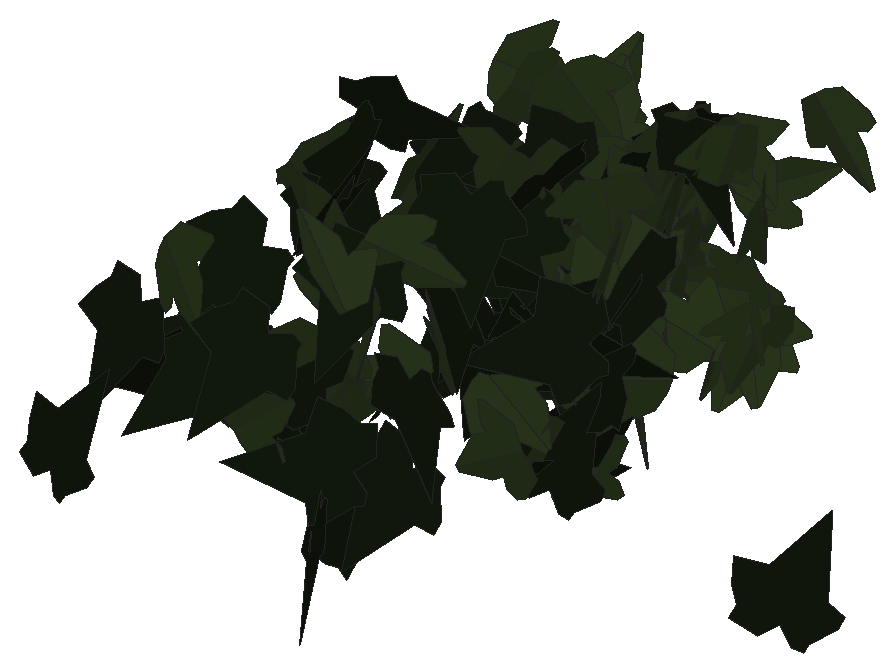
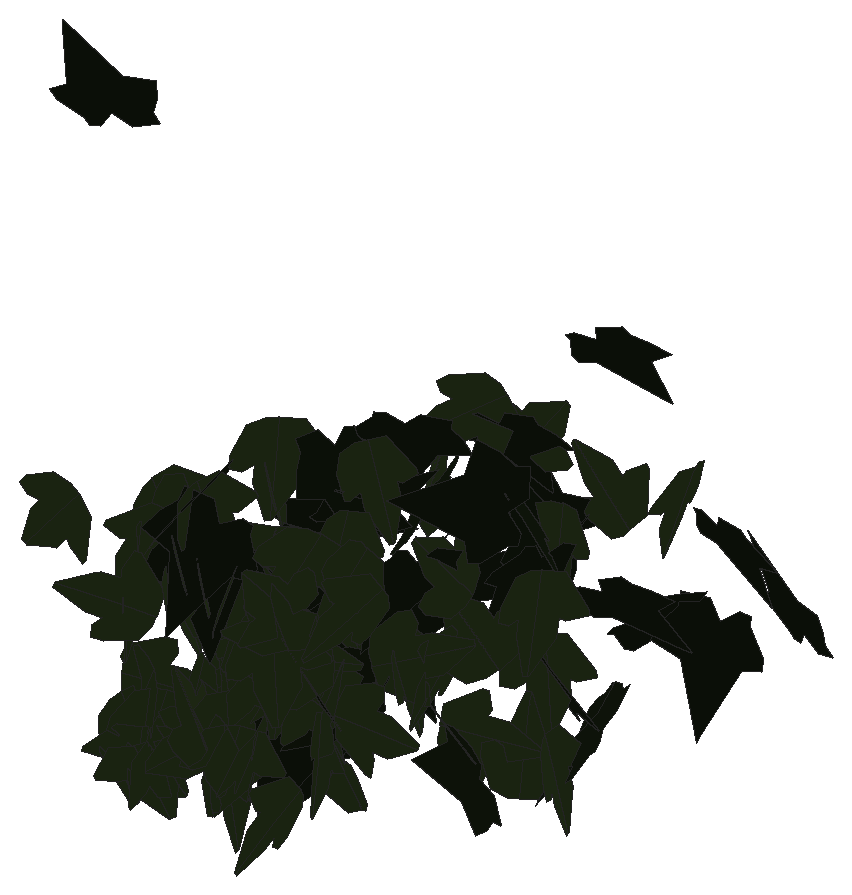
# SketchUp Ruby script. Lengths in inches.
U = 1.inch
M = Sketchup.active_model
def pt(a) = Geom::Point3d.new(a.map { |v| v * U })
def face(e, loops, mat)
  f = e.add_face(loops[0].map { |a| pt(a) })
  loops[1..].each { |l| e.add_face(l.map { |a| pt(a) }).erase! }
  f.material = f.back_material = mat if mat
  f
end
# faces: each face lists its corners as indices into pts; further lists are holes
def faces(e, pts, list, mat = nil) = list.each { |f| face(e, (f[0].is_a?(Array) ? f : [f]).map { |l| l.map { |i| pts[i] } }, mat) }
# xy, xz, yz: faces in a plane at the given z, y or x. An outline is a flat list of corners, or four numbers for a rectangle; further outlines are holes
def ring(l) = l.size == 4 ? [[l[0], l[1]], [l[2], l[1]], [l[2], l[3]], [l[0], l[3]]] : l.each_slice(2).to_a
def flat(e, list, mat, &to3) = list.each { |f| face(e, (f[0].is_a?(Array) ? f : [f]).map { |l| ring(l).map { |u, v| to3.(u, v) } }, mat) }
def xy(e, z, list, mat = nil) = flat(e, list, mat) { |x, y| [x, y, z] }
def xz(e, y, list, mat = nil) = flat(e, list, mat) { |x, z| [x, y, z] }
def yz(e, x, list, mat = nil) = flat(e, list, mat) { |y, z| [x, y, z] }
def lines(e, pts, list) = list.each { |a, b| e.add_line(pt(pts[a]), pt(pts[b])) }
# prism: a flat outline (further loops are holes) pulled along v
def prism(e, loops, v, mat = nil)
  f = face(e, loops, mat); d = Geom::Vector3d.new(v.map { |x| x * U })
  f.pushpull(f.normal.samedirection?(d) ? d.length : -d.length)
end
def box(e, o, s, mat = nil) = prism(e, [[o, [o[0] + s[0], o[1], o[2]], [o[0] + s[0], o[1] + s[1], o[2]], [o[0], o[1] + s[1], o[2]]]], [0, 0, s[2]], mat)
def at(x, y, z, deg = 0) = Geom::Transformation.translation(pt([x, y, z])) * Geom::Transformation.rotation(ORIGIN, Z_AXIS, deg.degrees)
def axes(o, x, y, z) = Geom::Transformation.new([*x, 0, *y, 0, *z, 0, *pt(o).to_a, 1])
def part(name) = M.definitions.add(name)
# library, detail: a bought-in or finely detailed component or shape, given as its bounding box
def library(name, o, s) = part(name).tap { |d| box(d.entities, o, s) }
def detail(e, o, s) = box(e.add_group.entities, o, s)
def put(e, d, t, mat = nil) = e.add_instance(d, t).tap { |i| i.material = mat if mat }
def group(e, t, mat = nil) = e.add_group.tap { |g| g.transformation = t; g.material = mat if mat }.entities
root = M.entities
M.materials.add("efeu1").color = [18, 25, 13]
M.materials.add("efeu2").color = [43, 57, 29]
c1 = part("ivyleaf_9")
p = [[1.54,2.16,1.25],[1.36,2.04,1.19],[-0.21,0.99,0.68],[-0.71,1.11,0.82],[-0.85,0.86,0.67],[-0.8,0.17,0.21],
  [-0.9,-0.01,0.1],[-0.67,-0.16,-0.02],[-0.08,-0.08,-0.05],[-0.03,-0.6,-0.4],[0.65,-0.88,-0.66],[0.83,-0.6,-0.49],
  [1.29,-0.42,-0.43],[1.8125,-0.07,-0.26],[1.21,0.44,0.15]]
faces(c1.entities,p,[[0,1,2,3,4,5,6,7,8,9,10,11,12,13,14]],"efeu1")
c2 = part("ivyleaf_10")
p = [[0,0.5,-0.03],[-0.0625,2.02,-0.43],[-0.19,2.01,-0.46],[-0.54,1.05,-0.29],[-0.52,0.625,-0.18],[-0.83,0.76,-0.28],
  [-1.16,0.64,-0.33],[-1.15,0.33,-0.24],[-0.77,-0.39,0.02],[-0.3,-0.51,0.16],[0.04,-0.48,0.23],[-0.02,2.01,-0.4375],
  [-0.06,2.01,-0.43],[0.04,-0.49,0.23],[0.67,-0.49,0.14],[1.38,0.36,-0.2],[1.375,0.51,-0.24],[0.81,0.65,-0.19],
  [0.62,0.59,-0.15],[0.6,1.09,-0.28],[0.5,1.23,-0.31]]
faces(c2.entities,p,[[0,1,2,3,4,5,6,7,8,9,10],[11,12,0,13,14,15,16,17,18,19,20]],"efeu2")
put(root,c1,axes([49.83,220.07,199.77],[0.12912,0.483,0.00603],[0.00148,0.00585,-0.49996],[-0.48304,0.12913,0.00008]))
put(root,c1,axes([49.8,218.5,199.04],[-0.2546,0.27025,0.33487],[0.23135,-0.24211,0.37129],[0.36284,0.34401,-0.00176]))
put(root,c1,axes([50.16,219.6,200.78],[-0.4643,-0.06001,-0.17558],[0.17405,0.0231,-0.46816],[0.0643,-0.49585,-0.00056]))
put(root,c1,axes([50.32,221.6,200.71],[-0.46544,-0.17562,0.05027],[-0.04688,-0.01815,-0.49747],[0.17655,-0.46779,0.00043]))
put(root,c2,axes([50.2,223.05,201.41],[-0.19142,-0.44375,-0.12822],[0.05054,0.11785,-0.48328],[0.45913,-0.19798,-0.00027]))
put(root,c1,axes([50.01,222.11,199.17],[0.28745,-0.40331,0.06863],[0.0407,-0.05528,-0.49527],[0.40708,0.29032,0.00105]))
put(root,c2,axes([50.34,222.62,198.92],[0.14203,-0.47928,-0.01095],[-0.00097,0.01113,-0.49988],[0.4794,0.14201,0.00223]))
put(root,c1,axes([50.61,220.58,199.8],[-0.33182,-0.29561,0.22915],[-0.16759,-0.15634,-0.44438],[0.33438,-0.37171,0.00467]))
put(root,c2,axes([50.49,219.86,201.42],[-0.08114,0.48141,0.10798],[-0.02245,0.10571,-0.48818],[-0.49286,-0.08407,0.00446]))
put(root,c1,axes([50.46,221.7,198.88],[0.36181,-0.31025,-0.15113],[-0.1135,0.09979,-0.47661],[0.3259,0.37919,0.00179]))
put(root,c2,axes([50.92,221.82,201.56],[-0.48046,0.09662,0.09913],[-0.09918,0.00955,-0.48997],[-0.09658,-0.49048,0.00999]))
put(root,c2,axes([51.18,225.41,200.33],[0.02007,0.02626,-0.49891],[-0.48071,0.13699,-0.01213],[0.13605,0.48015,0.03074]))
put(root,c1,axes([50.73,222.39,201.37],[0.08627,-0.31944,-0.37485],[-0.05713,0.3715,-0.32973],[0.48918,0.09973,0.0276]))
put(root,c1,axes([51.34,221.54,199.29],[-0.2039,0.25943,0.37566],[-0.24727,0.2831,-0.32972],[-0.38377,-0.32024,0.01285]))
put(root,c2,axes([50.97,222.49,198.35],[-0.13108,-0.44159,-0.19445],[-0.03019,-0.1936,0.46001],[-0.48157,0.13234,0.02409]))
put(root,c1,axes([51.31,222.1,201.94],[-0.27402,0.35103,0.22735],[-0.12971,0.18707,-0.44518],[-0.3976,-0.30296,-0.01146]))
put(root,c2,axes([51.14,221.8,199.67],[-0.46547,-0.14906,0.10542],[-0.09986,-0.03382,-0.48876],[0.15284,-0.47606,0.00171]))
put(root,c2,axes([51.05,223.03,200.26],[-0.16527,-0.4207,0.21377],[0.07665,0.19956,0.452],[-0.46563,0.18217,-0.00147]))
put(root,c1,axes([51.18,223.05,198.49],[-0.2363,0.41411,-0.15057],[-0.07466,0.13076,0.47679],[0.43427,0.24782,0.00003]))
put(root,c1,axes([51,221.86,201.08],[0.10251,0.45027,0.19169],[-0.0451,-0.18633,0.46179],[0.4873,-0.11197,0.00241]))
put(root,c2,axes([51.58,222.86,198.9],[-0.05009,-0.04479,0.49546],[-0.37395,-0.32503,-0.06719],[0.3281,-0.37729,-0.00094]))
put(root,c2,axes([51.33,223.4,200.3125],[-0.07243,0.3156,0.38098],[-0.11769,0.363,-0.32308],[-0.48052,-0.13648,0.0217]))
put(root,c2,axes([51.63,224.09,200.43],[-0.13004,-0.02615,-0.48208],[-0.46061,-0.14287,0.132],[-0.14465,0.47844,0.01306]))
put(root,c2,axes([51.22,225.15,201.84],[0.05047,0.2666,0.41997],[0.06245,0.41539,-0.2712],[-0.49351,0.07983,0.00863]))
put(root,c1,axes([50.9375,222.84,202.1875],[0.31664,-0.01751,0.38657],[0.38562,-0.02732,-0.3171],[0.03222,0.49895,-0.0038]))
put(root,c2,axes([51.32,223.24,201.22],[0.08773,-0.41779,0.26031],[-0.01201,0.26251,0.42537],[-0.4921,-0.08089,0.03602]))
put(root,c2,axes([51.66,223.81,200.34],[0.12623,-0.48378,0.00485],[0.00638,-0.00335,-0.49995],[0.48376,0.12628,0.00532]))
put(root,c1,axes([51.53,223.8,201.64],[0.01888,-0.34292,-0.36339],[-0.02302,0.36267,-0.34343],[0.49911,0.0297,-0.00209]))
put(root,c2,axes([51.71,224.68,201.95],[-0.09338,-0.31917,-0.37338],[0.13475,0.34884,-0.33189],[0.47236,-0.16261,0.02087]))
put(root,c1,axes([51.93,222.82,198.98],[-0.42263,0.25098,-0.0916],[-0.08658,0.03352,0.4913],[0.25276,0.43114,0.01513]))
put(root,c1,axes([51.82,224.04,200.05],[0.34584,-0.26231,-0.24817],[-0.19427,0.1545,-0.43404],[0.30439,0.39664,0.00494]))
put(root,c2,axes([52.16,224.77,199.48],[0.06951,-0.36421,-0.33544],[-0.0585,0.33031,-0.37077],[0.49168,0.0908,0.00331]))
put(root,c2,axes([52.23,224.71,199.6],[-0.30563,0.37403,-0.12918],[-0.09194,0.09163,0.48286],[0.38488,0.31891,0.01277]))
put(root,c1,axes([52.53,224.875,200.42],[-0.20129,0.28216,0.36037],[-0.21352,0.29033,-0.34658],[-0.40483,-0.29342,0.00361]))
put(root,c1,axes([51.95,224.22,199.93],[0.48125,-0.12604,0.05007],[0.04842,-0.01275,-0.49749],[0.12669,0.48368,-0.00007]))
put(root,c2,axes([52.32,224.74,199.92],[0.21971,0.3102,-0.32482],[-0.18873,-0.26436,-0.38012],[-0.40756,0.28964,0.00092]))
put(root,c2,axes([52.01,224.46,198.63],[0.39271,-0.16968,-0.25883],[0.23644,-0.10533,0.42779],[-0.1997,-0.45838,-0.00249]))
put(root,c2,axes([52.27,225.39,198.76],[-0.02139,0.28352,0.41129],[-0.06302,0.40685,-0.28373],[-0.49555,-0.06397,0.01833]))
put(root,c2,axes([52.22,224.99,202.1],[-0.36842,-0.2439,-0.23405],[0.21322,0.10097,-0.44084],[0.26231,-0.42464,0.02961]))
put(root,c2,axes([52.22,225.42,201.5],[0.18234,0.31912,-0.33899],[0.16527,0.29598,0.36753],[0.43525,-0.24608,0.00245]))
put(root,c2,axes([52.44,225.42,200.94],[-0.39083,-0.30742,0.05243],[-0.04486,-0.02777,-0.49721],[0.30861,-0.39335,-0.00587]))
put(root,c1,axes([52.66,224.46,201.28],[-0.3068,-0.09838,0.38235],[-0.36216,-0.12269,-0.32216],[0.15721,-0.47463,0.00403]))
put(root,c2,axes([52.52,220.33,201.5],[0.40122,0.07911,0.28768],[-0.28197,-0.05708,0.40895],[0.09754,-0.49039,-0.00119]))
put(root,c2,axes([52.24,225.48,201.15],[0.43303,0.20641,-0.14099],[0.12739,0.06041,0.47971],[0.21507,-0.45138,-0.00028]))
put(root,c2,axes([52.13,219.08,200.12],[-0.33541,-0.05464,0.36676],[0.36192,0.05943,0.33983],[-0.08073,0.49344,-0.00031]))
put(root,c2,axes([52.05,225.15,200.76],[-0.02195,-0.00444,-0.4995],[0.49588,0.06003,-0.02232],[0.06016,-0.49636,0.00177]))
put(root,c2,axes([52.66,224.92,200.45],[-0.15387,-0.02605,0.47502],[-0.18033,-0.4588,-0.08357],[0.44024,-0.19703,0.13179]))
put(root,c2,axes([52.625,225.34,201.01],[0.29143,0.32878,-0.23868],[-0.17746,-0.16122,-0.43877],[-0.36548,0.34045,0.02272]))
put(root,c1,axes([52.76,222.84,200.13],[0.16078,0.23602,-0.41042],[-0.23172,-0.33875,-0.28558],[-0.41286,0.28204,0.00046]))
put(root,c2,axes([52.68,225.45,200.42],[0.14841,0.28139,-0.38574],[-0.16466,-0.349,-0.31794],[-0.44818,0.2214,-0.01093]))
put(root,c1,axes([52.72,220.61,201.76],[-0.42528,-0.23691,-0.11405],[0.09951,0.05572,-0.48682],[0.24338,-0.43677,-0.00024]))
put(root,c2,axes([52.91,222.94,202.22],[-0.43622,-0.06768,0.2348],[-0.23065,-0.04463,-0.44137],[0.0807,-0.49338,0.00771]))
put(root,c2,axes([52.7,223.69,201.64],[-0.08137,-0.45926,-0.18016],[0.11652,0.15954,-0.45931],[0.47938,-0.11674,0.08106]))
put(root,c2,axes([52.63,225.04,200.5],[-0.29292,-0.32749,-0.23864],[0.2242,0.1143,-0.43205],[0.33754,-0.36012,0.07989]))
put(root,c2,axes([52.71,225.5,199.47],[-0.06763,0.47614,-0.13682],[0.0215,-0.13513,-0.48091],[-0.49494,-0.07093,-0.0022]))
put(root,c2,axes([52.9375,223.59,200.91],[-0.36806,-0.29799,0.16041],[-0.11422,-0.1137,-0.47331],[0.31856,-0.38506,0.01562]))
put(root,c1,axes([52.97,218.41,201.87],[-0.45217,-0.21316,-0.01049],[0.00912,0.00526,-0.49989],[0.21322,-0.45226,-0.00087]))
put(root,c1,axes([52.7,224.44,200.83],[-0.03287,-0.43385,-0.24636],[0.04713,0.24309,-0.43438],[0.49669,-0.05177,0.02492]))
put(root,c2,axes([52.84,225.67,199.51],[-0.37627,-0.31171,-0.10609],[0.16113,-0.03381,-0.47212],[0.28715,-0.38948,0.1259]))
put(root,c1,axes([53.26,223.79,199.41],[-0.45531,-0.01101,0.20632],[-0.20627,-0.00469,-0.45545],[0.01196,-0.49986,-0.00027]))
put(root,c2,axes([52.91,225.12,200.78],[-0.00654,0.02929,0.4991],[0.10621,-0.48767,0.03001],[0.48855,0.10641,0.00016]))
put(root,c1,axes([53.09,219.77,198.79],[0.00935,-0.48676,0.11393],[0.00171,0.11398,0.48683],[-0.49991,-0.00872,0.00379]))
put(root,c2,axes([52.91,225.58,200.04],[0.25847,0.42481,-0.05229],[-0.0444,-0.03414,-0.49685],[-0.4257,0.26148,0.02008]))
put(root,c2,axes([53.05,220.26,201.29],[0.25794,-0.40269,-0.14597],[-0.06715,0.13027,-0.47804],[0.42303,0.26622,0.01313]))
put(root,c1,axes([53.35,219.46,199.8],[-0.25398,-0.05527,0.42713],[-0.41963,-0.07989,-0.25986],[0.09698,-0.49047,-0.00581]))
put(root,c2,axes([53.04,224.36,200.09],[-0.17822,-0.45097,-0.12192],[0.0806,0.09885,-0.48346],[0.46015,-0.19198,0.03747]))
put(root,c2,axes([53.125,225.4,198.97],[0.05217,-0.49505,-0.04694],[-0.00418,0.04676,-0.49779],[0.49725,0.05234,0.00074]))
put(root,c1,axes([53.41,222.8125,201.19],[-0.29765,-0.37953,-0.13177],[-0.06152,-0.119,0.48172],[-0.39701,0.30298,0.02415]))
put(root,c2,axes([52.9,220.7,202.04],[-0.22567,-0.11337,-0.43153],[0.40488,0.15117,-0.25144],[0.18748,-0.46292,0.02357]))
put(root,c1,axes([53.35,222.37,200],[0.11132,0.35107,-0.33817],[-0.0958,-0.32436,-0.36826],[-0.47794,0.14678,-0.00495]))
put(root,c2,axes([53.15,225.99,199.7],[0.17904,-0.46067,0.07566],[-0.02462,0.0716,0.49423],[-0.46619,-0.1807,0.00296]))
put(root,c1,axes([53.01,221.79,200.97],[0.09898,-0.41866,0.2548],[0.06462,-0.24653,-0.43017],[0.48583,0.11809,0.0053]))
put(root,c1,axes([53.15,221.95,202.1875],[-0.27162,-0.33796,-0.24902],[0.16844,0.18394,-0.43335],[0.38452,-0.3193,0.01393]))
put(root,c1,axes([53.45,222.93,202.18],[-0.12579,0.46041,-0.14901],[0.03494,-0.14492,-0.47726],[-0.48266,-0.13048,0.00429]))
put(root,c1,axes([53.21,222.81,199.58],[0.39852,0.15507,0.2591],[-0.2538,-0.06044,0.42654],[0.16361,-0.47149,0.03054]))
put(root,c1,axes([53.34,223.75,198.83],[0.17554,0.45753,0.09924],[0.03076,0.09449,-0.49003],[-0.46716,0.17814,0.00502]))
put(root,c1,axes([53.04,223.13,200.43],[0.28975,-0.39697,0.09195],[0.04449,-0.08133,-0.49133],[0.40505,0.29291,-0.01181]))
put(root,c2,axes([53.08,225.84,199.61],[-0.31953,-0.02333,-0.38387],[0.38344,0.01906,-0.32033],[0.02958,-0.49909,0.00571]))
put(root,c1,axes([53.4,220.52,199.34],[-0.22036,-0.4147,0.17165],[-0.08668,-0.1483,-0.46957],[0.44037,-0.23671,-0.00653]))
put(root,c2,axes([53.26,222.31,199.61],[0.19727,0.35516,0.29146],[0.1334,0.25925,-0.4062],[-0.43965,0.23802,0.00753]))
put(root,c2,axes([53.53,221.03,200.57],[-0.37647,0.32903,-0.00235],[-0.00705,-0.0045,0.49993],[0.32896,0.37645,0.00803]))
put(root,c1,axes([53.36,218.92,199.42],[-0.26828,0.08747,-0.41277],[0.39866,-0.10767,-0.28192],[-0.1382,-0.48037,-0.01197]))
put(root,c2,axes([53.45,225.11,200.84],[-0.18705,-0.46162,-0.04383],[-0.01673,-0.04051,0.49808],[-0.46339,0.18779,-0.00029]))
put(root,c1,axes([53.26,220.73,200.34],[0.13652,-0.47457,0.07839],[0.02962,-0.07304,-0.49375],[0.48009,0.13946,0.00817]))
put(root,c2,axes([53.3,225.26,199.69],[-0.09316,0.17999,-0.45708],[0.22347,-0.39878,-0.20258],[-0.43747,-0.24203,-0.00615]))
put(root,c1,axes([53.69,222.87,200.24],[0.23423,0.04499,0.43945],[-0.43702,-0.04897,0.23795],[0.06445,-0.49556,0.01638]))
put(root,c2,axes([53.59,225.33,200.04],[0.07623,-0.33216,-0.36587],[0.00495,0.37069,-0.33551],[0.49413,0.04753,0.05981]))
put(root,c2,axes([53.69,223.75,198.99],[-0.08465,-0.37539,0.31924],[-0.06543,-0.31249,-0.3848],[0.48842,-0.10693,0.00378]))
put(root,c2,axes([53.42,225.16,200.78],[-0.06576,0.00923,0.49557],[0.3053,-0.39307,0.04783],[0.39047,0.30889,0.04606]))
put(root,c1,axes([53.79,224.96,201.68],[0.24035,0.37495,-0.22725],[-0.18918,-0.1451,-0.43949],[-0.39553,0.29725,0.07212]))
put(root,c1,axes([53.66,224.97,201.93],[0.28016,0.4133,0.02636],[0.01697,0.02034,-0.4993],[-0.41379,0.28066,-0.00263]))
put(root,c2,axes([53.59,222.96,198.48],[-0.00623,-0.27583,0.41699],[0.06752,0.41274,0.27403],[-0.49538,0.05973,0.0321]))
put(root,c2,axes([53.65,224.27,198.95],[-0.28618,0.39943,-0.09251],[0.04834,-0.07916,-0.49132],[-0.40714,-0.29015,0.00669]))
put(root,c1,axes([53.47,223.15,198.07],[0.29947,0.40018,0.01326],[-0.00972,-0.00929,0.49982],[0.40028,-0.29962,0.00221]))
put(root,c2,axes([54.09,221.54,199.37],[-0.24307,-0.00134,0.43694],[-0.43373,-0.0597,-0.24148],[0.05282,-0.49642,0.02786]))
put(root,c2,axes([53.77,225.04,201.375],[0.2281,-0.44241,0.04738],[0.03748,-0.03395,-0.49744],[0.44336,0.23048,0.01767]))
put(root,c2,axes([53.54,223.49,198.1875],[-0.34809,-0.10068,0.34453],[0.34608,0.03317,0.35935],[-0.09521,0.48863,0.0466]))
put(root,c1,axes([53.6875,222.77,198.28],[-0.31976,0.12633,0.36304],[0.31059,-0.19331,0.34083],[0.22647,0.44348,0.04515]))
put(root,c2,axes([53.99,225.01,199.33],[0.11674,0.30885,0.37548],[-0.1736,-0.33422,0.32888],[0.45413,-0.20716,0.0292]))
put(root,c2,axes([53.91,224.88,202.16],[-0.09455,-0.48398,0.08261],[-0.03313,-0.07765,-0.49282],[0.48986,-0.09867,-0.01739]))
put(root,c2,axes([53.9,225.92,199.17],[-0.04775,0.41865,-0.26918],[-0.13913,-0.27086,-0.39658],[-0.47787,0.03702,0.14236]))
put(root,c2,axes([53.86,223.66,201.12],[0.2958,0.38575,0.11704],[0.07067,0.0933,-0.48611],[-0.39687,0.30413,0.00068]))
put(root,c1,axes([54.23,223.7,200.8125],[-0.31874,0.38425,-0.02744],[0.02331,-0.01632,-0.49919],[-0.38453,-0.3195,-0.00751]))
put(root,c1,axes([53.58,223.23,199.91],[0.28175,-0.09209,0.40266],[0.38052,-0.13175,-0.29639],[0.16069,0.47346,-0.00416]))
put(root,c2,axes([54.38,225.48,199.85],[0.03053,0.03717,-0.49768],[-0.49888,0.01584,-0.02942],[0.01358,0.49837,0.03805]))
put(root,c2,axes([54.07,225.2,201.17],[0.11338,-0.48286,0.06319],[-0.00351,-0.06569,-0.49565],[0.48696,0.11195,-0.01828]))
put(root,c2,axes([54.01,225.625,199.5625],[-0.34552,-0.32884,-0.14994],[0.12717,0.08354,-0.47629],[0.3383,-0.36727,0.02591]))
put(root,c2,axes([54.04,225.93,199.04],[0.41993,0.23288,-0.13937],[-0.11307,-0.08331,-0.47987],[-0.24673,0.43454,-0.01731]))
put(root,c1,axes([54.45,223.06,199.85],[-0.22197,0.00471,-0.448],[-0.44803,-0.00115,0.22197],[0.00106,0.49998,0.00474]))
put(root,c2,axes([54.05,225.19,201.65],[0.26132,-0.4211,0.06623],[0.04318,-0.05113,-0.4955],[0.42408,0.26469,0.00965]))
put(root,c2,axes([54.18,223.95,199.31],[0.026,0.14464,0.47792],[-0.07579,-0.47187,0.14694],[0.49354,-0.08008,-0.00261]))
put(root,c1,axes([54.45,222.41,200.56],[-0.3103,-0.11691,0.37423],[-0.3519,-0.12737,-0.33157],[0.17286,-0.46916,-0.00323]))
put(root,c2,axes([54.21,223.11,202.15],[-0.34067,-0.36351,-0.04242],[0.04242,0.01835,-0.49786],[0.36351,-0.34281,0.01834]))
put(root,c1,axes([54.55,223.56,200.84],[-0.41034,0.21512,0.18802],[-0.17898,0.06292,-0.46261],[-0.22269,-0.44695,0.02537]))
put(root,c2,axes([54.12,225.84,199.22],[0.35209,0.3506,0.05577],[0.04034,0.03852,-0.49688],[-0.35271,0.35439,-0.00116]))
put(root,c1,axes([54.03,224.89,202.1875],[0.1938,-0.45347,-0.08254],[-0.01018,0.0853,-0.49256],[0.4608,0.19259,0.02383]))
put(root,c2,axes([54.4,225.13,201.99],[0.01611,0.35528,-0.35145],[-0.1711,-0.32646,-0.33786],[-0.46954,0.13115,0.11106]))
put(root,c2,axes([54.44,225.67,199.42],[-0.17549,-0.43841,0.16432],[-0.05755,-0.15396,-0.47221],[0.46464,-0.18465,0.00358]))
put(root,c2,axes([54.22,225.65,199.9375],[-0.35579,0.25301,-0.24372],[0.14577,-0.20929,-0.43006],[-0.31963,-0.37707,0.07516]))
put(root,c2,axes([54.3,225.25,201.84],[0.18534,0.37007,0.28052],[0.06721,0.27748,-0.41047],[-0.45949,0.18986,0.05311]))
put(root,c2,axes([54.46,222.92,201.62],[0.24196,-0.43624,-0.03392],[-0.01056,0.03293,-0.4988],[0.43743,0.2421,0.00672]))
put(root,c2,axes([54.51,224.99,202.07],[-0.09554,-0.4638,0.16052],[0.03562,-0.16965,-0.46899],[0.48949,-0.07817,0.06546]))
put(root,c2,axes([54.23,225.82,200.99],[-0.11564,-0.14673,0.46379],[0.29542,0.35755,0.18678],[-0.38646,0.31722,0.004]))
put(root,c2,axes([54.62,225.4,201.1],[0.15256,-0.44168,-0.17788],[0.01599,0.19143,-0.46162],[0.47589,0.13516,0.07254]))
put(root,c2,axes([55.12,226.07,202.23],[-0.39065,0.04998,-0.30805],[0.28825,-0.13139,-0.38685],[-0.11962,-0.47983,0.07384]))
put(root,c1,axes([61.4375,217.3,201.63],[-0.34555,0.04848,0.35812],[0.34827,-0.08759,0.3479],[0.09646,0.48988,0.02676]))
